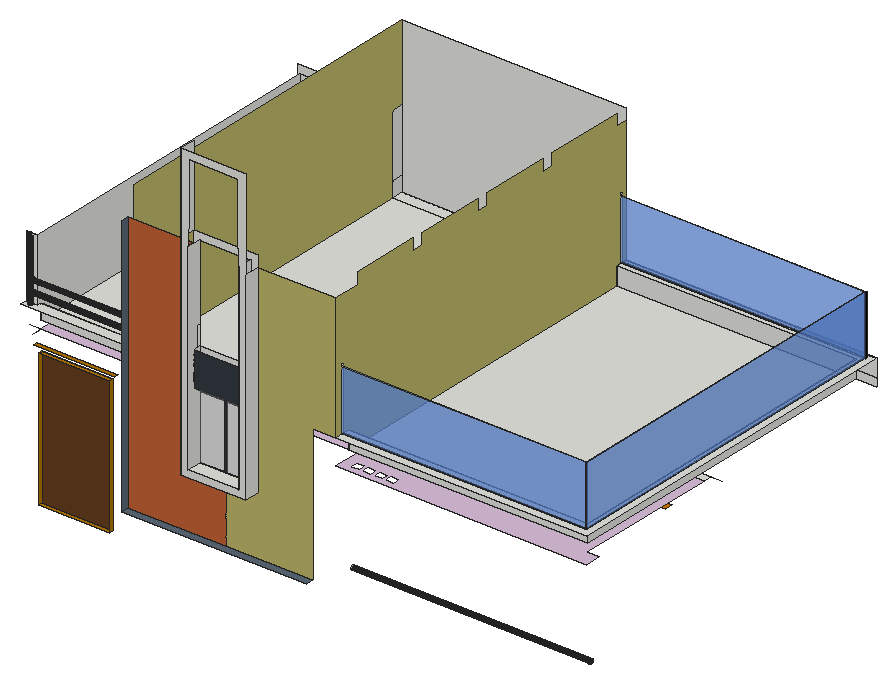
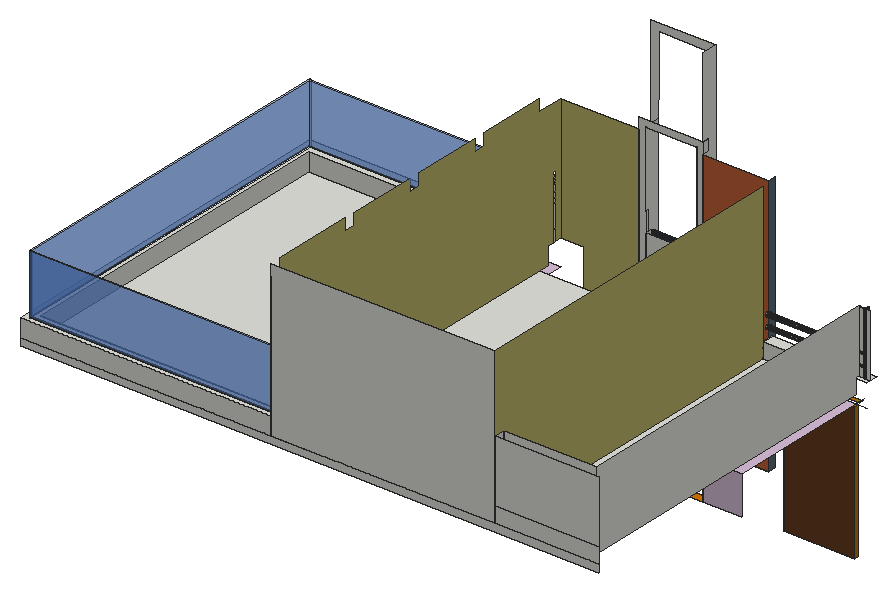
# SketchUp Ruby script. Lengths in inches.
U = 1.inch
M = Sketchup.active_model
def pt(a) = Geom::Point3d.new(a.map { |v| v * U })
def face(e, loops, mat)
  f = e.add_face(loops[0].map { |a| pt(a) })
  loops[1..].each { |l| e.add_face(l.map { |a| pt(a) }).erase! }
  f.material = f.back_material = mat if mat
  f
end
# faces: each face lists its corners as indices into pts; further lists are holes
def faces(e, pts, list, mat = nil) = list.each { |f| face(e, (f[0].is_a?(Array) ? f : [f]).map { |l| l.map { |i| pts[i] } }, mat) }
# xy, xz, yz: faces in a plane at the given z, y or x. An outline is a flat list of corners, or four numbers for a rectangle; further outlines are holes
def ring(l) = l.size == 4 ? [[l[0], l[1]], [l[2], l[1]], [l[2], l[3]], [l[0], l[3]]] : l.each_slice(2).to_a
def flat(e, list, mat, &to3) = list.each { |f| face(e, (f[0].is_a?(Array) ? f : [f]).map { |l| ring(l).map { |u, v| to3.(u, v) } }, mat) }
def xy(e, z, list, mat = nil) = flat(e, list, mat) { |x, y| [x, y, z] }
def xz(e, y, list, mat = nil) = flat(e, list, mat) { |x, z| [x, y, z] }
def yz(e, x, list, mat = nil) = flat(e, list, mat) { |y, z| [x, y, z] }
def lines(e, pts, list) = list.each { |a, b| e.add_line(pt(pts[a]), pt(pts[b])) }
# prism: a flat outline (further loops are holes) pulled along v
def prism(e, loops, v, mat = nil)
  f = face(e, loops, mat); d = Geom::Vector3d.new(v.map { |x| x * U })
  f.pushpull(f.normal.samedirection?(d) ? d.length : -d.length)
end
def box(e, o, s, mat = nil) = prism(e, [[o, [o[0] + s[0], o[1], o[2]], [o[0] + s[0], o[1] + s[1], o[2]], [o[0], o[1] + s[1], o[2]]]], [0, 0, s[2]], mat)
def at(x, y, z, deg = 0) = Geom::Transformation.translation(pt([x, y, z])) * Geom::Transformation.rotation(ORIGIN, Z_AXIS, deg.degrees)
def axes(o, x, y, z) = Geom::Transformation.new([*x, 0, *y, 0, *z, 0, *pt(o).to_a, 1])
def part(name) = M.definitions.add(name)
# library, detail: a bought-in or finely detailed component or shape, given as its bounding box
def library(name, o, s) = part(name).tap { |d| box(d.entities, o, s) }
def detail(e, o, s) = box(e.add_group.entities, o, s)
def put(e, d, t, mat = nil) = e.add_instance(d, t).tap { |i| i.material = mat if mat }
def group(e, t, mat = nil) = e.add_group.tap { |g| g.transformation = t; g.material = mat if mat }.entities
root = M.entities
M.materials.add("[0038_Orange]").color = [181, 117, 0]
M.materials.add("[0039_DarkOrange]").color = [214, 117, 0]
M.materials.add("[0057_DarkKhaki]").color = [188, 182, 106]
M.materials.add("[0111_SlateGray]").color = [51, 58, 66]
M.materials.add("[0111_SlateGray]1").color = [91, 104, 117]
M.materials.add("[0118_Thistle]").color = [216, 191, 216]
M.materials.add("[0137_Black]").color = [0, 0, 0]
M.materials.add("[Cladding Siding Tan]").color = [193, 97, 54]
M.materials.add("[Diamond Stripes]").color = [102, 61, 31]
M.materials.add("[Translucent Glass Blue]").color = [101, 150, 239]
M.materials["[Translucent Glass Blue]"].alpha = 0.5
M.materials.add("[Translucent Glass Gray]").color = [128, 128, 128]
M.materials["[Translucent Glass Gray]"].alpha = 0.5
xy(root,346.96,[[34.007,132,143.548,138]],"[0038_Orange]")
xy(root,404.14,[[186,102,474,114]],"[0111_SlateGray]1")
xy(root,438.843,[[554.676,378,633.073,380]])
xy(root,496.541,[[288.843,90,388.781,114]])
xy(root,506.882,[[299.183,90,378.44,114]])
xy(root,516,[[78,366,822,378]],"[0039_DarkOrange]")
xy(root,558.688,[[34.007,132,143.548,138]],"[0038_Orange]")
xy(root,567.511,[[25.184,132,152.371,138]],"[0038_Orange]")
xy(root,576,[[555.746,175.025,554.495,175.14,553.263,175.384,552.063,175.756,550.909,176.252,549.813,176.865,548.787,177.59,547.842,178.418,546.989,179.34,546.238,180.346,545.595,181.425,545.069,182.566,544.665,183.755,544.387,184.98,544.239,186.227,544.222,187.483,544.337,188.734,544.581,189.966,544.953,191.166,545.449,192.32,546.062,193.416,546.787,194.442,547.615,195.387,548.537,196.239,549.543,196.991,550.622,197.634,551.763,198.16,552.952,198.564,554.177,198.842,555.424,198.99,556.68,199.007,557.931,198.892,559.163,198.648,560.363,198.276,561.517,197.78,562.613,197.167,563.639,196.442,564.584,195.614,565.437,194.692,566.188,193.686,566.831,192.607,567.357,191.466,567.761,190.277,568.039,189.052,568.187,187.805,568.204,186.549,568.089,185.298,567.845,184.066,567.473,182.866,566.977,181.712,566.364,180.616,565.639,179.59,564.811,178.645,563.889,177.792,562.883,177.041,561.804,176.398,560.663,175.872,559.474,175.468,558.249,175.19,557.002,175.042],[689.058,175.025,687.808,175.14,686.576,175.384,685.376,175.756,684.222,176.252,683.126,176.865,682.1,177.59,681.155,178.418,680.302,179.34,679.55,180.346,678.908,181.425,678.381,182.566,677.977,183.755,677.7,184.98,677.551,186.227,677.535,187.483,677.649,188.734,677.894,189.966,678.266,191.166,678.761,192.32,679.375,193.416,680.099,194.442,680.927,195.387,681.849,196.239,682.855,196.991,683.935,197.634,685.075,198.16,686.264,198.564,687.489,198.842,688.737,198.99,689.993,199.007,691.243,198.892,692.476,198.648,693.675,198.276,694.829,197.78,695.926,197.167,696.952,196.442,697.896,195.614,698.749,194.692,699.501,193.686,700.144,192.607,700.67,191.466,701.074,190.277,701.352,189.052,701.5,187.805,701.516,186.549,701.402,185.298,701.157,184.066,700.785,182.866,700.29,181.712,699.676,180.616,698.952,179.59,698.124,178.645,697.202,177.792,696.196,177.041,695.116,176.398,693.976,175.872,692.787,175.468,691.562,175.19,690.314,175.042],[823.933,175.025,822.683,175.14,821.451,175.384,820.251,175.756,819.097,176.252,818.001,176.865,816.975,177.59,816.03,178.418,815.177,179.34,814.425,180.346,813.783,181.425,813.256,182.566,812.852,183.755,812.575,184.98,812.426,186.227,812.41,187.483,812.524,188.734,812.769,189.966,813.141,191.166,813.636,192.32,814.25,193.416,814.974,194.442,815.802,195.387,816.724,196.239,817.73,196.991,818.81,197.634,819.95,198.16,821.139,198.564,822.364,198.842,823.612,198.99,824.868,199.007,826.118,198.892,827.351,198.648,828.55,198.276,829.704,197.78,830.801,197.167,831.827,196.442,832.771,195.614,833.624,194.692,834.376,193.686,835.019,192.607,835.545,191.466,835.949,190.277,836.227,189.052,836.375,187.805,836.391,186.549,836.277,185.298,836.032,184.066,835.66,182.866,835.165,181.712,834.551,180.616,833.827,179.59,832.999,178.645,832.077,177.792,831.071,177.041,829.991,176.398,828.851,175.872,827.662,175.468,826.437,175.19,825.189,175.042],[78,366,882,378]])
xy(root,576,[[[510,114,510,156,18,156,18,378,78,378,78,366,882,366,882,138,900,138,900,114],[555.746,175.025,557.002,175.042,558.249,175.19,559.474,175.468,560.663,175.872,561.804,176.398,562.883,177.041,563.889,177.792,564.811,178.645,565.639,179.59,566.364,180.616,566.977,181.712,567.473,182.866,567.845,184.066,568.089,185.298,568.204,186.549,568.187,187.805,568.039,189.052,567.761,190.277,567.357,191.466,566.831,192.607,566.188,193.686,565.437,194.692,564.584,195.614,563.639,196.442,562.613,197.167,561.517,197.78,560.363,198.276,559.163,198.648,557.931,198.892,556.68,199.007,555.424,198.99,554.177,198.842,552.952,198.564,551.763,198.16,550.622,197.634,549.543,196.991,548.537,196.239,547.615,195.387,546.787,194.442,546.062,193.416,545.449,192.32,544.953,191.166,544.581,189.966,544.337,188.734,544.222,187.483,544.239,186.227,544.387,184.98,544.665,183.755,545.069,182.566,545.595,181.425,546.238,180.346,546.989,179.34,547.842,178.418,548.787,177.59,549.813,176.865,550.909,176.252,552.063,175.756,553.263,175.384,554.495,175.14],[689.058,175.025,690.314,175.042,691.562,175.19,692.787,175.468,693.976,175.872,695.116,176.398,696.196,177.041,697.202,177.792,698.124,178.645,698.952,179.59,699.676,180.616,700.29,181.712,700.785,182.866,701.157,184.066,701.402,185.298,701.516,186.549,701.5,187.805,701.352,189.052,701.074,190.277,700.67,191.466,700.144,192.607,699.501,193.686,698.749,194.692,697.896,195.614,696.952,196.442,695.926,197.167,694.829,197.78,693.675,198.276,692.476,198.648,691.243,198.892,689.993,199.007,688.737,198.99,687.489,198.842,686.264,198.564,685.075,198.16,683.935,197.634,682.855,196.991,681.849,196.239,680.927,195.387,680.099,194.442,679.375,193.416,678.761,192.32,678.266,191.166,677.894,189.966,677.649,188.734,677.535,187.483,677.551,186.227,677.7,184.98,677.977,183.755,678.381,182.566,678.908,181.425,679.55,180.346,680.302,179.34,681.155,178.418,682.1,177.59,683.126,176.865,684.222,176.252,685.376,175.756,686.576,175.384,687.808,175.14],[823.933,175.025,825.189,175.042,826.437,175.19,827.662,175.468,828.851,175.872,829.991,176.398,831.071,177.041,832.077,177.792,832.999,178.645,833.827,179.59,834.551,180.616,835.165,181.712,835.66,182.866,836.032,184.066,836.277,185.298,836.391,186.549,836.375,187.805,836.227,189.052,835.949,190.277,835.545,191.466,835.019,192.607,834.376,193.686,833.624,194.692,832.771,195.614,831.827,196.442,830.801,197.167,829.704,197.78,828.55,198.276,827.351,198.648,826.118,198.892,824.868,199.007,823.612,198.99,822.364,198.842,821.139,198.564,819.95,198.16,818.81,197.634,817.73,196.991,816.724,196.239,815.802,195.387,814.974,194.442,814.25,193.416,813.636,192.32,813.141,191.166,812.769,189.966,812.524,188.734,812.41,187.483,812.426,186.227,812.575,184.98,812.852,183.755,813.256,182.566,813.783,181.425,814.425,180.346,815.177,179.34,816.03,178.418,816.975,177.59,818.001,176.865,819.097,176.252,820.251,175.756,821.451,175.384,822.683,175.14],[524.459,124.289,538.647,136.289],[542.459,124.289,556.647,136.289],[560.459,124.289,574.647,136.289],[578.459,124.289,592.647,136.289]]],"[0118_Thistle]")
xy(root,588,[[510,139,882,660],[18,156,162,660],[162,156,510,660],[162,660,510,678]])
xy(root,612,[[0,138,162,138,162,156,18,156,18,149.683,10.283,149.683,10.653,149.504,11.245,148.991,11.683,148.342,11.939,147.602,11.995,146.82,11.846,146.051,11.504,145.347,10.991,144.755,10.342,144.317,9.602,144.061,8.82,144.005,8.051,144.154,7.347,144.496,6.755,145.009,6.317,145.658,6.061,146.398,6.005,147.18,6.154,147.949,6.496,148.653,7.009,149.245,7.658,149.683,0,149.683],[0,149.683,7.658,149.683,8.398,149.939,9.18,149.995,9.949,149.846,10.283,149.683,18,149.683,18,156,0,156],[7.658,149.683,8.398,149.939,9.18,149.995,9.949,149.846,10.283,149.683]])
xy(root,615.875,[[510,114,900,114,900,678,510,678,510,671,891,671,891,126.5,510,126.5],[510,126.5,889,128.5],[889,126.5,891,669],[510,128.5,889,128.5,889,669,510,669,510,660,882,660,882,139,510,139],[510,669,891,671]])
xy(root,616.285,[[299.183,102,378.44,114]],"[0111_SlateGray]")
xz(root,90,[[[288.843,496.541,388.781,951.916],[299.183,506.882,299.183,817.66,300.193,867.663,300.193,940.566,377.43,940.566,377.43,867.663,378.44,817.66,378.44,506.882]]])
xz(root,102,[[299.183,616.285,378.44,669.072]],"[0111_SlateGray]")
xz(root,114,[[[288.843,496.541,388.781,828],[299.183,506.882,378.44,817.66]],[299.183,616.285,378.44,669.072]])
xz(root,114,[[338.812,404.14,474,404.14,474,615.875,510,615.875,510,810,388.781,810,388.781,496.541,338.812,496.541]],"[0057_DarkKhaki]")
xz(root,114,[[337.435,506.882,340.694,616.285]],"[0111_SlateGray]")
xz(root,114,[[186,404.14,338.812,404.14,338.812,496.541,288.843,496.541,288.843,810,186,810]],"[Cladding Siding Tan]")
xz(root,114,[[299.183,506.882,337.435,616.285],[340.694,506.882,378.44,616.285]],"[Translucent Glass Gray]")
xz(root,126.5,[[889,615.875,891,708.875]],"[0137_Black]")
xz(root,126.5,[[510,615.875,889,708.875]],"[Translucent Glass Blue]")
xz(root,128.5,[[510,615.875,889,708.875]],"[Translucent Glass Blue]")
xz(root,138,[[34.007,346.96,143.548,558.688]],"[Diamond Stripes]")
xz(root,139,[[510,588,882,615.875]])
xz(root,149.683,[[0,612,7.658,612,7.658,709.342,18,709.342,18,709.653,0,709.653],[7.658,612,18,709.342]])
xz(root,156,[[18,588,162,612]])
xz(root,378,[[18,516,78,576]],"[0118_Thistle]")
xz(root,660,[[18,588,162,612],[510,588,882,615.875],[18,612,162,709.653]])
xz(root,669,[[889,615.875,891,708.875]])
xz(root,669,[[510,615.875,889,708.875]],"[Translucent Glass Blue]")
xz(root,671,[[510,615.875,891,708.875]],"[Translucent Glass Blue]")
xz(root,678,[[0,576,900,588],[0,588,162,612],[162,588,510,828],[510,588,900,615.875],[0,612,162,709.653]])
yz(root,9,[[147,625.835,146.799,625.862,147,625.861],[147,625.835,147,625.861,147.189,625.86],[147.575,625.911,147.952,626.01,147.776,625.9375],[146.412,625.913,146.224,625.9375,146.036,626.015],[148.3125,626.159,148.651,626.353,148.5,626.237],
  [145.676,626.164,145.5,626.237,145.339,626.361],[148.96,626.59,149.237,626.865,149.121,626.714],[145.03,626.598,144.879,626.714,144.755,626.875],[149.475,627.174,149.671,627.511,149.598,627.335],[144.518,627.184,144.402,627.335,144.324,627.523],
  [149.82,627.871,149.923,628.248,149.898,628.059],[144.175,627.883,144.102,628.059,144.076,628.26],[149.974,628.634,149.975,629.024,150,628.835],[144.025,628.646,144,628.835,144.026,629.036],[149.924,629.411,149.825,629.788,149.898,629.612],
  [144.077,629.423,144.102,629.612,144.18,629.799],[149.676,630.148,149.482,630.486,149.598,630.335],[144.329,630.159,144.402,630.335,144.525,630.496],[149.245,630.796,148.97,631.072,149.121,630.956],[144.763,630.805,144.879,630.956,145.04,631.08],
  [148.661,631.31,148.324,631.506,148.5,631.433],[145.349,631.317,145.5,631.433,145.6875,631.511],[147.964,631.655,147.588,631.758,147.776,631.733],[146.048,631.66,146.224,631.733,146.425,631.759],[147.201,631.809,147,631.81,147,631.835],
  [146.811,631.81,147,631.835,147,631.81],[147,643.48,146.98,643.483,147,643.485],[147,643.48,147,643.485,147.369,643.528],[146.592,643.534,146.224,643.582,146.205,643.59],[147.756,643.58,148.12,643.724,147.776,643.582],
  [145.843,643.74,145.5,643.882,145.484,643.894],[148.481,643.874,148.795,644.108,148.5,643.882],[145.174,644.132,144.879,644.359,144.866,644.375],[149.105,644.346,149.348,644.654,149.121,644.359],[144.628,644.685,144.402,644.98,144.394,644.999],
  [149.586,644.964,149.74,645.323,149.598,644.98],[144.244,645.36,144.102,645.703,144.1,645.724],[149.89,645.685,149.946,646.072,149.898,645.703],[144.049,646.111,144,646.48,144.003,646.5],[149.997,646.46,149.951,646.848,150,646.48],
  [144.054,646.888,144.102,647.256,144.11,647.275],[149.9,647.236,149.756,647.6,149.898,647.256],[144.26,647.637,144.402,647.98,144.414,647.996],[149.606,647.961,149.372,648.275,149.598,647.98],[144.652,648.306,144.879,648.601,144.895,648.614],
  [149.134,648.585,148.826,648.828,149.121,648.601],[145.205,648.852,145.5,649.078,145.519,649.086],[148.516,649.066,148.157,649.22,148.5,649.078],[145.88,649.235,146.224,649.378,146.244,649.38],[147.795,649.37,147.408,649.426,147.776,649.378],
  [146.631,649.431,147,649.48,147,649.475],[147,649.475,147,649.48,147.02,649.477]])
yz(root,18,[[156,588,660,588,660,709.653,149.683,709.653,149.683,612,156,612]])
yz(root,34.007,[[132,346.96,138,558.688]],"[0038_Orange]")
yz(root,78,[[366,516,378,576]])
yz(root,143.548,[[132,346.96,138,558.688]],"[0038_Orange]")
yz(root,162,[[138,588,156,612],[660,588,678,612],[660,612,678,709.653],[147.379,625.859,147,625.861,146.596,625.862,145.84,626.068,145.164,626.463,144.612,627.019,144.224,627.699,144.024,628.456,144.027,629.239,144.233,629.995,144.628,630.671,145.184,631.223,145.863,631.612,146.621,631.811,147,631.81,147.404,631.808,148.16,631.602,148.836,631.208,149.388,630.652,149.776,629.972,149.976,629.214,149.973,628.431,149.767,627.676,149.372,626.999,148.816,626.448,148.137,626.059],[146.96,643.48,146.185,643.593,145.465,643.902,144.851,644.387,144.382,645.015,144.092,645.742,144,646.52,144.113,647.295,144.422,648.015,144.907,648.629,145.535,649.098,146.262,649.388,147,649.475,147.04,649.48,147.815,649.367,148.535,649.058,149.149,648.573,149.618,647.945,149.908,647.218,150,646.44,149.887,645.665,149.578,644.945,149.093,644.33,148.465,643.862,147.738,643.572,147,643.485]])
yz(root,162,[[156,588,156,828,678,828,678,709.653,660,709.653,660,588]],"[0057_DarkKhaki]")
yz(root,186,[[102,404.14,114,810]],"[0111_SlateGray]1")
yz(root,288.843,[[90,496.541,90,951.916,114,951.916,114,828,102,828,102,810,114,810,114,496.541]])
yz(root,299.183,[[90,506.882,114,506.882,114,616.285,102,616.285,102,669.072,108,669.072,108,700.424,114,700.424,114,817.66,90,817.66],[102,616.285,114,669.072]])
yz(root,378.44,[[90,506.882,90,817.66,114,817.66,114,700.424,108,700.424,108,669.072,102,669.072,102,616.285,114,616.285,114,506.882],[102,616.285,114,669.072]])
yz(root,388.781,[[90,496.541,114,810]])
yz(root,510,[[147,417,146.224,417.102,145.5,417.402,144.879,417.879,144.402,418.5,144.102,419.224,144,420,144.102,420.776,144.402,421.5,144.879,422.121,145.5,422.598,146.224,422.898,147,423,147.776,422.898,148.5,422.598,149.121,422.121,149.598,421.5,149.898,420.776,150,420,149.898,419.224,149.598,418.5,149.121,417.879,148.5,417.402,147.776,417.102],[660,588,678,615.875],[126.5,615.875,128.5,708.875],[669,615.875,671,708.875]])
yz(root,510,[[[139,588,660,588,660,615.875,678,615.875,678,810,660,810,660,828,534,828,534,810,516,810,516,828,408,828,408,810,390,810,390,828,282,828,282,810,264,810,264,828,156,828,156,810,114,810,114,615.875,126.5,615.875,126.5,708.875,125.724,708.977,125,709.277,124.379,709.754,123.902,710.375,123.602,711.099,123.5,711.875,123.602,712.651,123.902,713.375,124.379,713.996,125,714.473,125.724,714.773,126.5,714.875,127.276,714.773,128,714.473,128.621,713.996,129.098,713.375,129.398,712.651,129.5,711.875,129.398,711.099,129.098,710.375,128.621,709.754,128,709.277,127.276,708.977,126.5,708.875,128.5,708.875,128.5,615.875,139,615.875],[669,708.875,668.224,708.977,667.5,709.277,666.879,709.754,666.402,710.375,666.102,711.099,666,711.875,666.102,712.651,666.402,713.375,666.879,713.996,667.5,714.473,668.224,714.773,669,714.875,669.776,714.773,670.5,714.473,671.121,713.996,671.598,713.375,671.898,712.651,672,711.875,671.898,711.099,671.598,710.375,671.121,709.754,670.5,709.277,669.776,708.977]]],"[0057_DarkKhaki]")
yz(root,882,[[139,588,660,615.875]])
yz(root,889,[[126.5,615.875,128.5,708.875]])
yz(root,889,[[128.5,615.875,669,708.875]],"[Translucent Glass Blue]")
yz(root,891,[[669,615.875,671,708.875]],"[0137_Black]")
yz(root,891,[[126.5,615.875,669,708.875]],"[Translucent Glass Blue]")
p = [[510,146.224,417.102],[510,147,417],[882,147,417],[882,146.224,417.102],[510,147.776,417.102],[882,147.776,417.102],
  [510,145.5,417.402],[882,145.5,417.402],[510,148.5,417.402],[882,148.5,417.402],[510,144.879,417.879],[882,144.879,417.879],
  [510,149.121,417.879],[882,149.121,417.879],[510,144.402,418.5],[882,144.402,418.5],[510,149.598,418.5],[882,149.598,418.5],
  [510,144.102,419.224],[882,144.102,419.224],[510,149.898,419.224],[882,149.898,419.224],[510,144,420],[882,144,420],
  [510,150,420],[882,150,420],[510,144.102,420.776],[882,144.102,420.776],[510,149.898,420.776],[882,149.898,420.776],
  [510,144.402,421.5],[882,144.402,421.5],[510,149.598,421.5],[882,149.598,421.5],[510,144.879,422.121],[882,144.879,422.121],
  [510,149.121,422.121],[882,149.121,422.121],[510,145.5,422.598],[882,145.5,422.598],[510,148.5,422.598],[882,148.5,422.598],
  [510,146.224,422.898],[882,146.224,422.898],[510,147.776,422.898],[882,147.776,422.898],[510,147,423],[882,147,423],
  [8.82,144.005,708.18],[8.051,144.154,708.949],[8.051,144.154,612],[8.82,144.005,612],[9.602,144.061,707.398],[9.602,144.061,612],
  [10.342,144.317,706.658],[10.342,144.317,612],[7.347,144.496,709.653],[7.347,144.496,612],[10.991,144.755,706.009],[10.991,144.755,612],
  [6.755,145.009,710.245],[6.755,145.009,612],[11.504,145.347,705.496],[11.504,145.347,612],[6.317,145.658,710.683],[6.317,145.658,612],
  [11.846,146.051,705.154],[11.846,146.051,612],[6.061,146.398,710.939],[6.061,146.398,612],[11.995,146.82,705.005],[11.995,146.82,612],
  [6.005,147.18,710.995],[6.005,147.18,612],[11.939,147.602,705.061],[11.982,147,705.018],[11.939,147.602,612],[6.154,147.949,710.846],
  [6.154,147.949,612],[11.683,148.342,705.317],[11.683,148.342,612],[6.496,148.653,710.504],[6.496,148.653,612],[11.245,148.991,705.755],
  [11.245,148.991,612],[7.009,149.245,709.991],[7.009,149.245,612],[10.653,149.504,706.347],[10.653,149.504,612],[7.658,149.683,709.342],
  [7.658,149.683,612],[9.949,149.846,707.051],[10.283,149.683,612],[9.949,149.846,612],[8.398,149.939,708.602],[8.398,149.939,612],
  [9.18,149.995,707.82],[9.18,149.995,612],[162,145.84,626.068],[162,146.596,625.862],[9,146.596,625.862],[9,146.412,625.913],
  [9,146.036,626.015],[9,145.84,626.068],[162,147,625.861],[162,147.379,625.859],[9,147.379,625.859],[9,147.189,625.86],
  [9,147,625.861],[9,146.799,625.862],[162,148.137,626.059],[9,148.137,626.059],[9,147.952,626.01],[9,147.575,625.911],
  [162,145.164,626.463],[9,145.676,626.164],[9,145.339,626.361],[9,145.164,626.463],[162,148.816,626.448],[9,148.816,626.448],
  [9,148.651,626.353],[9,148.3125,626.159],[162,149.372,626.999],[9,149.372,626.999],[9,149.237,626.865],[9,148.96,626.59],
  [162,144.612,627.019],[9,145.03,626.598],[9,144.755,626.875],[9,144.612,627.019],[162,144.224,627.699],[9,144.518,627.184],
  [9,144.324,627.523],[9,144.224,627.699],[162,149.767,627.676],[9,149.767,627.676],[9,149.671,627.511],[9,149.475,627.174],
  [162,144.024,628.456],[9,144.175,627.883],[9,144.076,628.26],[9,144.024,628.456],[162,149.973,628.431],[9,149.973,628.431],
  [9,149.923,628.248],[9,149.82,627.871],[162,149.976,629.214],[9,149.976,629.214],[9,149.975,629.024],[9,149.974,628.634],
  [162,144.027,629.239],[9,144.025,628.646],[9,144.026,629.036],[9,144.027,629.239],[162,144.233,629.995],[9,144.077,629.423],
  [9,144.18,629.799],[9,144.233,629.995],[162,149.776,629.972],[9,149.776,629.972],[9,149.825,629.788],[9,149.924,629.411],
  [162,144.628,630.671],[9,144.329,630.159],[9,144.525,630.496],[9,144.628,630.671],[162,149.388,630.652],[9,149.388,630.652],
  [9,149.482,630.486],[9,149.676,630.148],[162,145.184,631.223],[9,144.763,630.805],[9,145.04,631.08],[9,145.184,631.223],
  [162,148.836,631.208],[9,148.836,631.208],[9,148.97,631.072],[9,149.245,630.796],[162,145.863,631.612],[9,145.349,631.317],
  [9,145.6875,631.511],[9,145.863,631.612],[162,148.16,631.602],[9,148.16,631.602],[9,148.324,631.506],[9,148.661,631.31],
  [162,146.621,631.811],[9,146.048,631.66],[9,146.425,631.759],[9,146.621,631.811],[162,147.404,631.808],[9,147.404,631.808],
  [9,147.588,631.758],[9,147.964,631.655],[162,147,631.81],[9,146.811,631.81],[9,147,631.81],[9,147.201,631.809],
  [162,146.185,643.593],[162,146.96,643.48],[9,146.96,643.48],[9,146.592,643.534],[9,146.205,643.59],[9,146.185,643.593],
  [162,147,643.485],[162,147.738,643.572],[9,147.738,643.572],[9,147.369,643.528],[9,147,643.485],[9,146.98,643.483],
  [162,145.465,643.902],[9,145.843,643.74],[9,145.484,643.894],[9,145.465,643.902],[162,148.465,643.862],[9,148.465,643.862],
  [9,148.12,643.724],[9,147.756,643.58],[162,144.851,644.387],[9,145.174,644.132],[9,144.866,644.375],[9,144.851,644.387],
  [162,149.093,644.33],[9,149.093,644.33],[9,148.795,644.108],[9,148.481,643.874],[162,149.578,644.945],[9,149.578,644.945],
  [9,149.348,644.654],[9,149.105,644.346],[162,144.382,645.015],[9,144.628,644.685],[9,144.394,644.999],[9,144.382,645.015],
  [162,149.887,645.665],[9,149.887,645.665],[9,149.74,645.323],[9,149.586,644.964],[162,144.092,645.742],[9,144.244,645.36],
  [9,144.1,645.724],[9,144.092,645.742],[162,144,646.52],[9,144.049,646.111],[9,144.003,646.5],[9,144,646.52],
  [162,150,646.44],[9,150,646.44],[9,149.946,646.072],[9,149.89,645.685],[162,149.908,647.218],[9,149.908,647.218],
  [9,149.951,646.848],[9,149.997,646.46],[162,144.113,647.295],[9,144.054,646.888],[9,144.11,647.275],[9,144.113,647.295],
  [162,149.618,647.945],[9,149.618,647.945],[9,149.756,647.6],[9,149.9,647.236],[162,144.422,648.015],[9,144.26,647.637],
  [9,144.414,647.996],[9,144.422,648.015],[162,149.149,648.573],[9,149.149,648.573],[9,149.372,648.275],[9,149.606,647.961],
  [162,144.907,648.629],[9,144.652,648.306],[9,144.895,648.614],[9,144.907,648.629],[162,145.535,649.098],[9,145.205,648.852],
  [9,145.519,649.086],[9,145.535,649.098],[162,148.535,649.058],[9,148.535,649.058],[9,148.826,648.828],[9,149.134,648.585],
  [162,146.262,649.388],[9,145.88,649.235],[9,146.244,649.38],[9,146.262,649.388],[162,147.815,649.367],[9,147.815,649.367],
  [9,148.157,649.22],[9,148.516,649.066],[162,147,649.475],[9,146.631,649.431],[9,147,649.475],[9,147.02,649.477],
  [9,147.04,649.48],[162,147.04,649.48],[9,147.408,649.426],[9,147.795,649.37],[882,378,576],[900,378,576],
  [18,156,576],[0,156,576],[18,138,576],[9,147,612],[9,147,625.835],[9,147,628.835],
  [162,147,628.835],[9,147,646.48],[162,147,646.48],[9,147,649.48],[9,147,660.682],[9,147,631.835],
  [9,147,643.48],[882,147,420],[510,147,420]]
faces(root,p,[[0,1,2,3],[1,4,5,2],[6,0,3,7],[4,8,9,5],[10,6,7,11],[8,12,13,9],[14,10,11,15],[12,16,17,13],
  [18,14,15,19],[16,20,21,17],[22,18,19,23],[20,24,25,21],[26,22,23,27],[24,28,29,25],[30,26,27,31],[28,32,33,29],
  [34,30,31,35],[32,36,37,33],[38,34,35,39],[36,40,41,37],[42,38,39,43],[40,44,45,41],[46,42,43,47],[44,46,47,45]],"[0137_Black]")
faces(root,p,[[48,49,50,51],[52,48,51,53],[54,52,53,55],[49,56,57,50],[58,54,55,59],[56,60,61,57],[62,58,59,63],[60,64,65,61],
  [66,62,63,67],[64,68,69,65],[70,66,67,71],[68,72,73,69],[74,75,70,71,76],[72,77,78,73],[79,74,76,80],[77,81,82,78],
  [83,79,80,84],[81,85,86,82],[87,83,84,88],[85,89,90,86],[91,87,88,92,93],[89,94,95,90],[96,91,93,97],[94,96,97,95],
  [98,99,100,101,102,103],[99,104,105,106,107,108,109,100],[105,110,111,112,113,106],[114,98,103,115,116,117],[110,118,119,120,121,111],[118,122,123,124,125,119],[126,114,117,127,128,129],[130,126,129,131,132,133],
  [122,134,135,136,137,123],[138,130,133,139,140,141],[134,142,143,144,145,135],[142,146,147,148,149,143],[150,138,141,151,152,153],[154,150,153,155,156,157],[146,158,159,160,161,147],[162,154,157,163,164,165],
  [158,166,167,168,169,159],[170,162,165,171,172,173],[166,174,175,176,177,167],[178,170,173,179,180,181],[174,182,183,184,185,175],[186,178,181,187,188,189],[182,190,191,192,193,183],[194,186,189,195,196,197,191,190],
  [198,199,200,201,202,203],[204,205,206,207,208,209,200,199],[210,198,203,211,212,213],[205,214,215,216,217,206],[218,210,213,219,220,221],[214,222,223,224,225,215],[222,226,227,228,229,223],[230,218,221,231,232,233],
  [226,234,235,236,237,227],[238,230,233,239,240,241],[242,238,241,243,244,245],[234,246,247,248,249,235],[246,250,251,252,253,247],[254,242,245,255,256,257],[250,258,259,260,261,251],[262,254,257,263,264,265],
  [258,266,267,268,269,259],[270,262,265,271,272,273],[274,270,273,275,276,277],[266,278,279,280,281,267],[282,274,277,283,284,285],[278,286,287,288,289,279],[290,282,285,291,292,293,294,295],[286,295,294,296,297,287]])
lines(root,p,[[298,299],[300,301],[300,302],[303,304],[305,306],[307,308],[309,310],[311,312],[313,314],[314,1],[2,313]])
